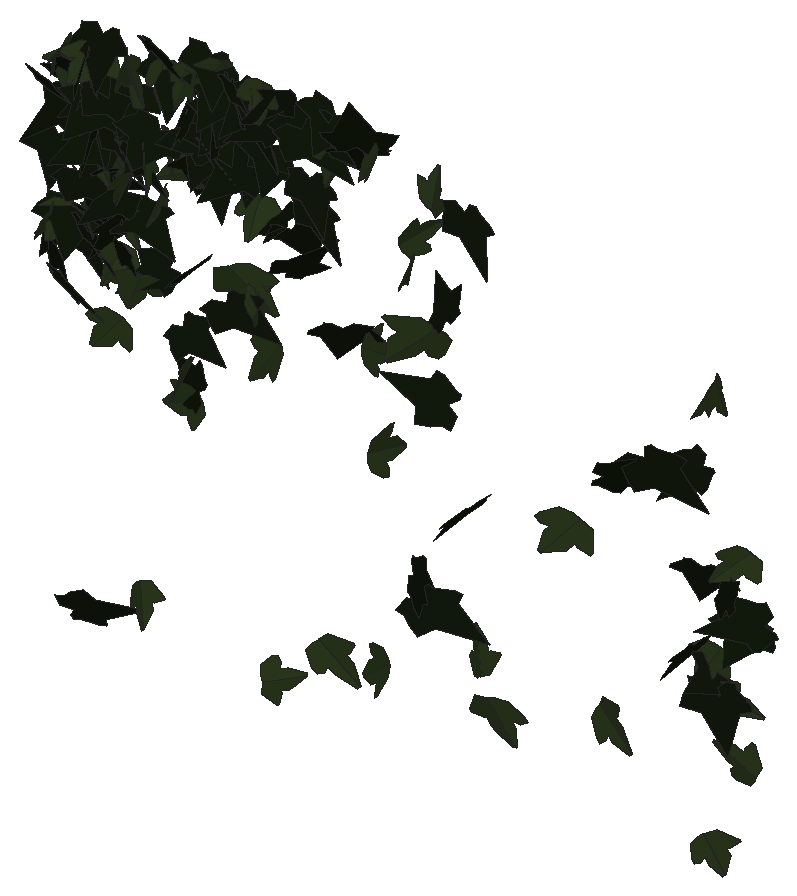
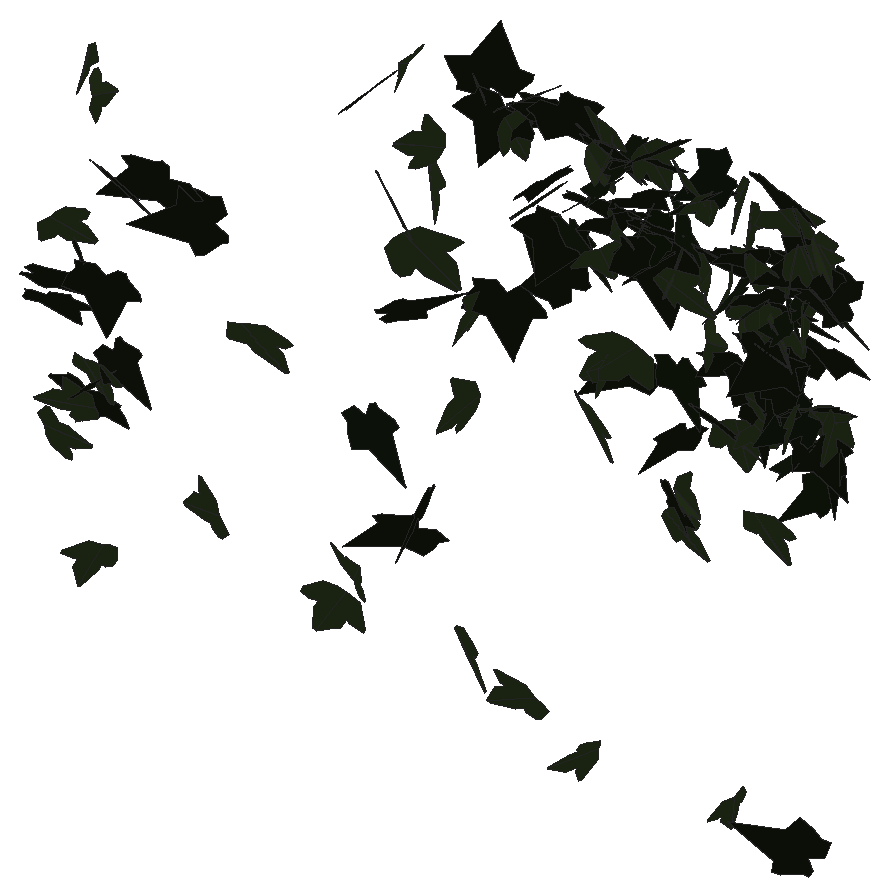
# SketchUp Ruby script. Lengths in inches.
U = 1.inch
M = Sketchup.active_model
def pt(a) = Geom::Point3d.new(a.map { |v| v * U })
def face(e, loops, mat)
  f = e.add_face(loops[0].map { |a| pt(a) })
  loops[1..].each { |l| e.add_face(l.map { |a| pt(a) }).erase! }
  f.material = f.back_material = mat if mat
  f
end
# faces: each face lists its corners as indices into pts; further lists are holes
def faces(e, pts, list, mat = nil) = list.each { |f| face(e, (f[0].is_a?(Array) ? f : [f]).map { |l| l.map { |i| pts[i] } }, mat) }
# xy, xz, yz: faces in a plane at the given z, y or x. An outline is a flat list of corners, or four numbers for a rectangle; further outlines are holes
def ring(l) = l.size == 4 ? [[l[0], l[1]], [l[2], l[1]], [l[2], l[3]], [l[0], l[3]]] : l.each_slice(2).to_a
def flat(e, list, mat, &to3) = list.each { |f| face(e, (f[0].is_a?(Array) ? f : [f]).map { |l| ring(l).map { |u, v| to3.(u, v) } }, mat) }
def xy(e, z, list, mat = nil) = flat(e, list, mat) { |x, y| [x, y, z] }
def xz(e, y, list, mat = nil) = flat(e, list, mat) { |x, z| [x, y, z] }
def yz(e, x, list, mat = nil) = flat(e, list, mat) { |y, z| [x, y, z] }
def lines(e, pts, list) = list.each { |a, b| e.add_line(pt(pts[a]), pt(pts[b])) }
# prism: a flat outline (further loops are holes) pulled along v
def prism(e, loops, v, mat = nil)
  f = face(e, loops, mat); d = Geom::Vector3d.new(v.map { |x| x * U })
  f.pushpull(f.normal.samedirection?(d) ? d.length : -d.length)
end
def box(e, o, s, mat = nil) = prism(e, [[o, [o[0] + s[0], o[1], o[2]], [o[0] + s[0], o[1] + s[1], o[2]], [o[0], o[1] + s[1], o[2]]]], [0, 0, s[2]], mat)
def at(x, y, z, deg = 0) = Geom::Transformation.translation(pt([x, y, z])) * Geom::Transformation.rotation(ORIGIN, Z_AXIS, deg.degrees)
def axes(o, x, y, z) = Geom::Transformation.new([*x, 0, *y, 0, *z, 0, *pt(o).to_a, 1])
def part(name) = M.definitions.add(name)
# library, detail: a bought-in or finely detailed component or shape, given as its bounding box
def library(name, o, s) = part(name).tap { |d| box(d.entities, o, s) }
def detail(e, o, s) = box(e.add_group.entities, o, s)
def put(e, d, t, mat = nil) = e.add_instance(d, t).tap { |i| i.material = mat if mat }
def group(e, t, mat = nil) = e.add_group.tap { |g| g.transformation = t; g.material = mat if mat }.entities
root = M.entities
M.materials.add("1026 AP 7946 SUNNY SIDE UP").color = [254, 231, 186]
M.materials.add("efeu1").color = [18, 25, 13]
M.materials.add("efeu2").color = [43, 57, 29]
c1 = part("ivyleaf_9")
p = [[1.54,2.16,1.25],[1.36,2.04,1.19],[-0.21,0.99,0.68],[-0.71,1.11,0.82],[-0.85,0.86,0.67],[-0.8,0.17,0.21],
  [-0.9,-0.01,0.1],[-0.67,-0.16,-0.02],[-0.08,-0.08,-0.05],[-0.03,-0.6,-0.4],[0.65,-0.88,-0.66],[0.83,-0.6,-0.49],
  [1.29,-0.42,-0.43],[1.8125,-0.07,-0.26],[1.21,0.44,0.15]]
faces(c1.entities,p,[[0,1,2,3,4,5,6,7,8,9,10,11,12,13,14]],"efeu1")
c2 = part("ivyleaf_10")
p = [[0,0.5,-0.03],[-0.0625,2.02,-0.43],[-0.19,2.01,-0.46],[-0.54,1.05,-0.29],[-0.52,0.625,-0.18],[-0.83,0.76,-0.28],
  [-1.16,0.64,-0.33],[-1.15,0.33,-0.24],[-0.77,-0.39,0.02],[-0.3,-0.51,0.16],[0.04,-0.48,0.23],[-0.02,2.01,-0.4375],
  [-0.06,2.01,-0.43],[0.04,-0.49,0.23],[0.67,-0.49,0.14],[1.38,0.36,-0.2],[1.375,0.51,-0.24],[0.81,0.65,-0.19],
  [0.62,0.59,-0.15],[0.6,1.09,-0.28],[0.5,1.23,-0.31]]
faces(c2.entities,p,[[0,1,2,3,4,5,6,7,8,9,10],[11,12,0,13,14,15,16,17,18,19,20]],"efeu2")
put(root,c1,axes([127.99,212.35,274.9],[0.2386,-0.046,-0.27535],[-0.41018,0.05791,-0.16266],[0.11515,0.30161,-0.00889]),"1026 AP 7946 SUNNY SIDE UP")
put(root,c1,axes([127.54,212.61,277.8],[0.30684,-0.18203,0.16089],[0.1912,-0.1,-0.27537],[0.32631,0.22977,0.01006]),"1026 AP 7946 SUNNY SIDE UP")
put(root,c2,axes([127.93,212.35,275.47],[-0.04301,-0.23789,-0.23167],[0.05468,0.22091,-0.2453],[0.51036,-0.04372,0.00676]),"1026 AP 7946 SUNNY SIDE UP")
put(root,c1,axes([128.04,212.64,275.1875],[0.00942,0.23509,-0.17942],[0.0038,-0.17557,-0.24323],[-0.46129,0.00335,-0.00567]),"1026 AP 7946 SUNNY SIDE UP")
put(root,c2,axes([127.98,212.68,278.6],[0.0953,-0.30672,0.00333],[-0.02376,-0.00805,-0.32169],[0.48176,0.06028,-0.01652]),"1026 AP 7946 SUNNY SIDE UP")
put(root,c1,axes([127.89,212.6,276.85],[-0.36333,-0.10161,-0.1693],[0.26317,0.02097,-0.25656],[0.15025,-0.28243,0.03998]),"1026 AP 7946 SUNNY SIDE UP")
put(root,c1,axes([128.22,212.48,277.72],[-0.48161,0.1498,-0.12186],[0.14484,-0.08171,-0.35027],[-0.26381,-0.31833,0.03016]),"1026 AP 7946 SUNNY SIDE UP")
put(root,c2,axes([128.18,212.78,278.42],[-0.26163,-0.24846,0.09229],[-0.01566,-0.10153,-0.30496],[0.41575,-0.16018,0.04659]),"1026 AP 7946 SUNNY SIDE UP")
put(root,c2,axes([128.22,212.47,275.59],[0.38077,0.12339,-0.11725],[-0.14542,-0.07012,-0.27972],[-0.22118,0.25852,-0.01794]),"1026 AP 7946 SUNNY SIDE UP")
put(root,c1,axes([128.08,212.38,274.3],[0.41901,-0.13176,-0.08034],[-0.0798,0.07011,-0.30318],[0.22651,0.26844,0.04181]),"1026 AP 7946 SUNNY SIDE UP")
put(root,c1,axes([127.98,212.57,278.25],[0.44552,0.04071,0.12678],[0.19072,0.0195,-0.29477],[-0.07091,0.3082,0.00374]),"1026 AP 7946 SUNNY SIDE UP")
put(root,c1,axes([128.28,212.52,275.62],[-0.25069,-0.24515,-0.04338],[0.06927,0.01973,-0.29996],[0.38457,-0.16336,0.02575]),"1026 AP 7946 SUNNY SIDE UP")
put(root,c2,axes([128.31,212.62,277.34],[0.11567,-0.29374,0.00492],[0.11757,0.01229,-0.30203],[0.44678,0.07281,0.0782]),"1026 AP 7946 SUNNY SIDE UP")
put(root,c1,axes([128.23,212.84,274.98],[0.17548,-0.27226,0.02357],[0.01504,-0.02248,-0.30326],[0.42956,0.11201,0.00099]),"1026 AP 7946 SUNNY SIDE UP")
put(root,c2,axes([128.53,212.64,278.29],[-0.25269,0.24743,0.11069],[-0.12618,0.07385,-0.30238],[-0.40404,-0.17781,0.02521]),"1026 AP 7946 SUNNY SIDE UP")
put(root,c2,axes([128.51,212.65,275.5625],[-0.16157,0.25366,0.11537],[-0.0912,0.09555,-0.28087],[-0.42542,-0.11683,0.0164]),"1026 AP 7946 SUNNY SIDE UP")
put(root,c1,axes([128.39,212.64,278.77],[-0.21028,0.01901,-0.29032],[0.40213,-0.12447,-0.13435],[-0.18891,-0.28612,0.03716]),"1026 AP 7946 SUNNY SIDE UP")
put(root,c1,axes([128.3125,212.62,275.57],[0.4558,-0.05076,-0.00583],[-0.01034,-0.00643,-0.30311],[0.0796,0.28985,-0.00599]),"1026 AP 7946 SUNNY SIDE UP")
put(root,c1,axes([128.37,212.87,277.28],[0.23794,-0.25749,0.05404],[0.04225,-0.04675,-0.30796],[0.4115,0.15369,0.00037]),"1026 AP 7946 SUNNY SIDE UP")
put(root,c2,axes([128.78,212.49,278.79],[0.40867,0.10648,-0.14054],[-0.18521,-0.07297,-0.289],[-0.20037,0.28461,-0.01951]),"1026 AP 7946 SUNNY SIDE UP")
put(root,c2,axes([128.78,212.74,276.96],[0.2219,-0.26805,-0.04438],[-0.05542,0.02833,-0.31137],[0.4229,0.14436,-0.01751]),"1026 AP 7946 SUNNY SIDE UP")
put(root,c1,axes([128.97,212.5,277.15],[-0.46108,-0.02133,0.05455],[-0.07729,-0.04777,-0.29985],[0.04599,-0.29414,0.04297]),"1026 AP 7946 SUNNY SIDE UP")
put(root,c1,axes([128.83,212.6,277.8125],[-0.33045,-0.19934,0.09583],[-0.05109,-0.10065,-0.29483],[0.34285,-0.20712,0.04843]),"1026 AP 7946 SUNNY SIDE UP")
put(root,c1,axes([128.6875,212.5625,277.375],[-0.22287,0.04578,-0.27231],[0.36202,-0.13325,-0.15159],[-0.21728,-0.26896,0.02675]),"1026 AP 7946 SUNNY SIDE UP")
put(root,c1,axes([128.39,212.52,267.93],[0.15057,-0.04342,0.2928],[0.45115,-0.00847,-0.10088],[0.03453,0.30003,0.04131]),"1026 AP 7946 SUNNY SIDE UP")
put(root,c1,axes([128.55,212.52,275.39],[0.24814,-0.24452,0.05174],[0.01895,-0.05352,-0.29951],[0.3925,0.15717,-0.01825]),"1026 AP 7946 SUNNY SIDE UP")
put(root,c1,axes([128.99,212.54,275.62],[0.16965,-0.14209,0.25963],[-0.22303,0.20943,0.18484],[-0.39776,-0.17804,0.00709]),"1026 AP 7946 SUNNY SIDE UP")
put(root,c1,axes([129.09,212.61,278.11],[-0.47798,0.00001,0.0364],[-0.05531,-0.02867,-0.31195],[0.00519,-0.30468,0.02756]),"1026 AP 7946 SUNNY SIDE UP")
put(root,c1,axes([128.62,212.34,276.51],[-0.02841,-0.10689,-0.29868],[0.17158,0.26886,-0.10777],[0.45362,-0.10839,0.02206]),"1026 AP 7946 SUNNY SIDE UP")
put(root,c2,axes([128.61,212.6,276.89],[0.28998,-0.06078,0.23919],[0.34699,-0.07328,-0.20046],[0.1497,0.28759,0.00133]),"1026 AP 7946 SUNNY SIDE UP")
put(root,c2,axes([129.01,212.75,273.56],[0.41792,-0.07395,-0.12679],[-0.18136,0.04276,-0.28379],[0.13351,0.28958,0.01137]),"1026 AP 7946 SUNNY SIDE UP")
put(root,c1,axes([128.77,212.52,276.375],[0.34241,0.21301,0.15905],[0.17709,0.1039,-0.31319],[-0.37261,0.24513,-0.00269]),"1026 AP 7946 SUNNY SIDE UP")
put(root,c1,axes([128.93,212.51,279.19],[-0.35687,-0.08126,-0.2231],[0.35704,-0.02377,-0.23661],[0.06564,-0.31248,0.07406]),"1026 AP 7946 SUNNY SIDE UP")
put(root,c1,axes([129.01,212.81,277.5],[-0.22148,-0.26899,-0.00087],[0.00897,-0.00376,-0.31275],[0.42286,-0.1408,0.00618]),"1026 AP 7946 SUNNY SIDE UP")
put(root,c2,axes([129.25,212.6,277.1],[-0.46009,-0.05613,0.03196],[-0.03464,-0.0497,-0.3038],[0.09497,-0.29005,0.04406]),"1026 AP 7946 SUNNY SIDE UP")
put(root,c2,axes([129.04,212.83,278.01],[0.44831,-0.06202,0.10589],[0.14973,-0.04594,-0.2999],[0.11573,0.29969,-0.02219]),"1026 AP 7946 SUNNY SIDE UP")
put(root,c1,axes([129.3,212.4375,275.36],[0.27622,-0.02047,-0.2536],[-0.38694,0.01002,-0.1818],[0.03154,0.30216,-0.00937]),"1026 AP 7946 SUNNY SIDE UP")
put(root,c2,axes([129.23,212.625,275.06],[0.1726,0.21273,-0.1807],[-0.12477,-0.1578,-0.24752],[-0.41646,0.13544,-0.00074]),"1026 AP 7946 SUNNY SIDE UP")
put(root,c1,axes([129.03,212.7,277.33],[0.16864,-0.29083,-0.02972],[0.00926,0.03112,-0.31871],[0.4592,0.10618,0.01734]),"1026 AP 7946 SUNNY SIDE UP")
put(root,c1,axes([129.44,212.48,276.35],[-0.46351,0.02819,-0.04096],[0.05495,-0.04903,-0.3018],[-0.05372,-0.2934,0.04472]),"1026 AP 7946 SUNNY SIDE UP")
put(root,c2,axes([129.3,212.625,278.71],[0.10779,-0.26987,-0.16559],[0.05505,0.16854,-0.27781],[0.48959,0.04046,0.06769]),"1026 AP 7946 SUNNY SIDE UP")
put(root,c1,axes([129.28,212.89,278.14],[-0.24342,-0.26367,0.00497],[0.02881,-0.01807,-0.31404],[0.41371,-0.15388,0.02479]),"1026 AP 7946 SUNNY SIDE UP")
put(root,c1,axes([129.47,212.42,275.87],[-0.08769,0.25781,-0.22566],[0.07086,-0.21586,-0.273],[-0.52872,-0.07169,0.00084]),"1026 AP 7946 SUNNY SIDE UP")
put(root,c2,axes([129.13,212.83,275.67],[0.1786,-0.03269,0.2821],[0.37532,-0.13707,-0.11958],[0.21777,0.26305,-0.02527]),"1026 AP 7946 SUNNY SIDE UP")
put(root,c2,axes([129.47,212.52,276.68],[0.02689,-0.30373,0.05021],[0.01116,-0.05014,-0.31366],[0.484,0.01803,0.00444]),"1026 AP 7946 SUNNY SIDE UP")
put(root,c2,axes([129.73,212.48,274.77],[-0.3898,-0.14838,0.07193],[-0.07288,-0.05958,-0.29673],[0.24793,-0.2508,0.02587]),"1026 AP 7946 SUNNY SIDE UP")
put(root,c2,axes([129.58,212.78,268.58],[0.06164,0.29237,-0.07784],[-0.0167,-0.07649,-0.30434],[-0.4752,0.04062,0.0006]),"1026 AP 7946 SUNNY SIDE UP")
put(root,c2,axes([129.73,212.34,278.84],[-0.21135,0.28741,0.08549],[-0.07828,0.0664,-0.32604],[-0.4631,-0.14239,0.0161]),"1026 AP 7946 SUNNY SIDE UP")
put(root,c1,axes([129.61,212.47,277.27],[0.28431,-0.2237,-0.12274],[-0.10458,0.09773,-0.29561],[0.38359,0.19245,0.01038]),"1026 AP 7946 SUNNY SIDE UP")
put(root,c1,axes([129.57,212.59,276.06],[-0.0612,-0.2065,-0.2284],[0.26236,0.17068,-0.19398],[0.39605,-0.14498,0.09321]),"1026 AP 7946 SUNNY SIDE UP")
put(root,c1,axes([130.14,212.74,275.02],[-0.45594,0.07886,-0.00566],[-0.00286,-0.02922,-0.30833],[-0.12432,-0.28855,0.02784]),"1026 AP 7946 SUNNY SIDE UP")
put(root,c2,axes([129.89,212.49,277.24],[-0.06175,0.23853,-0.20952],[0.05414,-0.20182,-0.25021],[-0.49129,-0.05222,-0.00124]),"1026 AP 7946 SUNNY SIDE UP")
put(root,c2,axes([130,212.82,276.35],[-0.08975,0.1631,-0.25348],[-0.06826,-0.25342,-0.16356],[-0.46035,0.00578,0.07367]),"1026 AP 7946 SUNNY SIDE UP")
put(root,c1,axes([130.09,212.55,277.73],[-0.40678,-0.15578,-0.01435],[0.03527,-0.01202,-0.31036],[0.24327,-0.25875,0.021]),"1026 AP 7946 SUNNY SIDE UP")
put(root,c1,axes([129.82,212.6875,279.23],[0.45135,-0.13655,0.00495],[-0.0128,-0.03004,-0.32612],[0.21451,0.28552,-0.02987]),"1026 AP 7946 SUNNY SIDE UP")
put(root,c2,axes([130.04,212.76,278.8],[0.14593,0.28498,-0.06993],[-0.01965,-0.06898,-0.30902],[-0.46082,0.09319,-0.00897]),"1026 AP 7946 SUNNY SIDE UP")
put(root,c2,axes([130.07,212.8,277.52],[-0.21283,0.2009,-0.18028],[0.08526,-0.17268,-0.24685],[-0.41137,-0.13973,0.04211]),"1026 AP 7946 SUNNY SIDE UP")
put(root,c1,axes([130.11,212.91,278.77],[-0.13353,-0.29427,0.02455],[0.00438,-0.02733,-0.31551],[0.46442,-0.08435,0.01004]),"1026 AP 7946 SUNNY SIDE UP")
put(root,c2,axes([130.74,212.85,277.1],[-0.24165,-0.05176,0.2626],[-0.34884,-0.12912,-0.16537],[0.21437,-0.26846,0.02692]),"1026 AP 7946 SUNNY SIDE UP")
put(root,c1,axes([130.61,212.5,277.88],[0.08769,0.08498,0.3436],[0.04648,0.33497,-0.09119],[-0.53847,0.04276,0.04808]),"1026 AP 7946 SUNNY SIDE UP")
put(root,c2,axes([130.59,212.68,278.91],[0.35705,-0.21916,0.01935],[-0.00182,-0.02997,-0.32447],[0.34603,0.22598,-0.02168]),"1026 AP 7946 SUNNY SIDE UP")
put(root,c2,axes([130.9,212.48,272.82],[0.23053,-0.09939,-0.25825],[-0.31554,0.14943,-0.18148],[0.28201,0.24844,0.00806]),"1026 AP 7946 SUNNY SIDE UP")
put(root,c2,axes([130.68,212.61,273.39],[0.16454,-0.23069,0.18315],[0.08703,-0.17113,-0.2614],[0.4509,0.11721,-0.01639]),"1026 AP 7946 SUNNY SIDE UP")
put(root,c1,axes([131.04,212.45,273.11],[-0.24552,0.11226,-0.24567],[-0.38367,0.0451,0.18623],[0.1591,0.28199,0.06997]),"1026 AP 7946 SUNNY SIDE UP")
put(root,c2,axes([130.72,212.86,277.03],[-0.14901,0.24243,0.15972],[0.10611,-0.13846,0.26711],[0.43866,0.11584,-0.01036]),"1026 AP 7946 SUNNY SIDE UP")
put(root,c1,axes([131.1,212.71,277.84],[-0.40482,0.08649,0.13841],[-0.2316,-0.03197,-0.27073],[-0.09573,-0.28841,0.06966]),"1026 AP 7946 SUNNY SIDE UP")
put(root,c1,axes([130.91,212.42,275.41],[-0.08129,0.29429,-0.03334],[0.01593,-0.03277,-0.30798],[-0.46555,-0.05251,-0.00472]),"1026 AP 7946 SUNNY SIDE UP")
put(root,c1,axes([131.0625,212.7,277.45],[0.2267,0.29437,-0.16466],[-0.09493,-0.15017,-0.33837],[-0.51935,0.15594,-0.01002]),"1026 AP 7946 SUNNY SIDE UP")
put(root,c1,axes([130.85,212.35,274.29],[0.10184,-0.16027,-0.25801],[-0.08016,0.2456,-0.17469],[0.45939,0.07838,0.02671]),"1026 AP 7946 SUNNY SIDE UP")
put(root,c2,axes([131.11,212.85,279.2],[-0.16476,-0.26485,0.11791],[-0.01694,-0.11967,-0.29233],[0.4543,-0.10051,0.03186]),"1026 AP 7946 SUNNY SIDE UP")
put(root,c1,axes([130.97,212.91,279.32],[-0.0851,-0.30283,0.03364],[0.0093,-0.03595,-0.31688],[0.47913,-0.05309,0.01212]),"1026 AP 7946 SUNNY SIDE UP")
put(root,c1,axes([131.13,212.6875,277.84],[-0.40091,-0.12565,-0.10832],[0.18875,-0.01276,-0.28618],[0.17428,-0.27523,0.06077]),"1026 AP 7946 SUNNY SIDE UP")
put(root,c1,axes([131.12,212.8125,277.25],[-0.01663,-0.30447,0.02122],[-0.00646,-0.0222,-0.31396],[0.47999,-0.01085,-0.00349]),"1026 AP 7946 SUNNY SIDE UP")
put(root,c1,axes([131.04,212.62,277.71],[0.38641,-0.19039,0.0366],[0.0205,-0.04274,-0.31942],[0.30417,0.24475,-0.02496]),"1026 AP 7946 SUNNY SIDE UP")
put(root,c1,axes([131.38,212.83,278.93],[-0.37233,-0.19213,0.00309],[0.02224,-0.0239,-0.313],[0.30136,-0.23561,0.02692]),"1026 AP 7946 SUNNY SIDE UP")
put(root,c1,axes([131.39,212.89,278.375],[-0.28893,-0.23198,0.07906],[-0.05144,-0.07346,-0.30465],[0.38141,-0.18564,0.01881]),"1026 AP 7946 SUNNY SIDE UP")
put(root,c1,axes([131.18,212.88,278.03],[0.13832,-0.11525,-0.27788],[0.31252,-0.18277,0.14651],[-0.33793,-0.2162,0.02175]),"1026 AP 7946 SUNNY SIDE UP")
put(root,c1,axes([131.51,212.82,278.98],[0.25183,-0.26002,0.02195],[0.0234,-0.01759,-0.31469],[0.40975,0.16081,0.00448]),"1026 AP 7946 SUNNY SIDE UP")
put(root,c1,axes([132.01,212.5,277.74],[-0.49214,-0.02006,-0.02789],[0.045,-0.0268,-0.32192],[0.02769,-0.313,0.0275]),"1026 AP 7946 SUNNY SIDE UP")
put(root,c2,axes([131.74,212.66,275.49],[-0.46413,-0.05384,-0.21885],[0.33845,-0.007,-0.30676],[0.06224,-0.36342,0.03616]),"1026 AP 7946 SUNNY SIDE UP")
put(root,c1,axes([132.08,212.78,278.97],[-0.47182,-0.02701,-0.06739],[0.10729,-0.03724,-0.30753],[0.0287,-0.30481,0.04172]),"1026 AP 7946 SUNNY SIDE UP")
put(root,c2,axes([131.72,212.82,277.6875],[0.3008,-0.08753,0.23033],[0.29151,-0.12879,-0.21564],[0.24105,0.26499,-0.02664]),"1026 AP 7946 SUNNY SIDE UP")
put(root,c1,axes([131.93,212.84,277.8],[-0.18788,-0.28286,-0.00493],[0.01204,0.00022,-0.31625],[0.44464,-0.11953,0.00648]),"1026 AP 7946 SUNNY SIDE UP")
put(root,c2,axes([131.93,212.8,278.98],[-0.0872,0.23128,-0.19637],[0.05168,-0.18933,-0.24593],[-0.46974,-0.06376,0.00939]),"1026 AP 7946 SUNNY SIDE UP")
put(root,c1,axes([131.81,212.32,275.1],[-0.00596,-0.10008,-0.29943],[0.11996,0.28069,-0.09915],[0.46737,-0.07332,0.02163]),"1026 AP 7946 SUNNY SIDE UP")
put(root,c1,axes([131.86,212.87,278.46],[0.18004,-0.27999,0.0594],[0.02411,-0.05772,-0.31187],[0.44936,0.11528,-0.00707]),"1026 AP 7946 SUNNY SIDE UP")
put(root,c2,axes([132.15,212.87,278.8],[0.04648,-0.28859,0.10377],[-0.0034,-0.10304,-0.29921],[0.48147,0.02713,-0.01213]),"1026 AP 7946 SUNNY SIDE UP")
put(root,c2,axes([132.19,212.53,275.02],[0.0439,0.10049,-0.30666],[0.0501,0.29697,0.10789],[0.49232,-0.03918,0.01637]),"1026 AP 7946 SUNNY SIDE UP")
put(root,c1,axes([132.22,212.86,278.03],[-0.40748,-0.15099,-0.06976],[0.14153,-0.02485,-0.30174],[0.21769,-0.26647,0.0656]),"1026 AP 7946 SUNNY SIDE UP")
put(root,c2,axes([132.21,212.625,277.03],[0.24233,0.23783,-0.12051],[-0.08248,-0.10686,-0.29227],[-0.40947,0.16228,-0.01244]),"1026 AP 7946 SUNNY SIDE UP")
put(root,c2,axes([132.22,212.63,279.23],[0.42788,-0.12238,0.077],[0.09836,-0.04462,-0.30727],[0.20353,0.27883,-0.01338]),"1026 AP 7946 SUNNY SIDE UP")
put(root,c2,axes([132.4375,212.69,274.27],[0.37718,-0.27248,-0.08313],[-0.11473,0.04091,-0.3727],[0.43115,0.24926,-0.02645]),"1026 AP 7946 SUNNY SIDE UP")
put(root,c1,axes([132.6875,212.45,278.89],[-0.42814,0.14758,-0.00802],[-0.00662,-0.02581,-0.3182],[-0.23235,-0.2712,0.02384]),"1026 AP 7946 SUNNY SIDE UP")
put(root,c1,axes([132.36,212.79,277.98],[-0.10995,-0.26936,0.13799],[-0.00382,-0.13857,-0.28592],[0.47408,-0.06359,0.0297]),"1026 AP 7946 SUNNY SIDE UP")
put(root,c1,axes([132.97,212.4,277.07],[-0.23451,0.26882,0.01624],[-0.03593,0.00358,-0.31612],[-0.42175,-0.14977,0.0179]),"1026 AP 7946 SUNNY SIDE UP")
put(root,c1,axes([133,212.61,279.24],[0.04097,0.08317,-0.30941],[-0.26756,-0.24926,-0.08764],[-0.4114,0.1704,0.02619]),"1026 AP 7946 SUNNY SIDE UP")
put(root,c2,axes([132.65,212.37,268.13],[0.08025,-0.06743,-0.31215],[0.24775,0.26978,-0.03297],[0.41986,-0.1463,0.07912]),"1026 AP 7946 SUNNY SIDE UP")
put(root,c1,axes([133.15,212.375,276.97],[0.37703,0.18975,-0.04615],[-0.02924,-0.05013,-0.31403],[-0.30556,0.23893,-0.02689]),"1026 AP 7946 SUNNY SIDE UP")
put(root,c1,axes([133,212.45,276.11],[0.3312,0.23716,0.03298],[-0.05768,-0.00834,0.32595],[0.37156,-0.21269,0.0212]),"1026 AP 7946 SUNNY SIDE UP")
put(root,c1,axes([133.32,212.62,277.875],[0.0185,-0.30912,-0.03279],[-0.01298,0.02977,-0.31843],[0.48819,0.0125,-0.00722]),"1026 AP 7946 SUNNY SIDE UP")
put(root,c1,axes([133.15,212.47,279.0625],[0.06575,-0.15404,-0.27872],[0.32008,0.2191,-0.09513],[0.36882,-0.16269,0.13225]),"1026 AP 7946 SUNNY SIDE UP")
put(root,c1,axes([133.43,212.54,277.49],[0.13045,-0.30943,-0.03813],[0.01305,0.03867,-0.32929],[0.48953,0.08143,0.01894]),"1026 AP 7946 SUNNY SIDE UP")
put(root,c1,axes([133.37,212.41,278.9375],[-0.00495,-0.20042,-0.24959],[0.24591,0.20801,-0.17899],[0.42733,-0.12202,0.10011]),"1026 AP 7946 SUNNY SIDE UP")
put(root,c1,axes([133.68,212.8,279.1875],[-0.20367,-0.24956,0.14229],[-0.00859,-0.151,-0.28432],[0.4495,-0.11596,0.05904]),"1026 AP 7946 SUNNY SIDE UP")
put(root,c2,axes([133.9,212.69,278.62],[-0.07107,-0.27731,0.14063],[0.05059,-0.14299,-0.28583],[0.48448,-0.02575,0.05048]),"1026 AP 7946 SUNNY SIDE UP")
put(root,c2,axes([133.6,212.6875,268.91],[0.28581,0.06099,0.26352],[0.40563,0.01684,-0.19314],[-0.0775,0.31307,-0.03905]),"1026 AP 7946 SUNNY SIDE UP")
put(root,c1,axes([134.14,212.58,278.79],[0.2912,0.25346,-0.00007],[0.01687,-0.0097,-0.32311],[-0.3982,0.18495,-0.01373]),"1026 AP 7946 SUNNY SIDE UP")
put(root,c1,axes([134.25,212.35,275.46],[0.23761,0.24629,-0.1335],[-0.10655,-0.1121,-0.29833],[-0.42549,0.16561,0.00015]),"1026 AP 7946 SUNNY SIDE UP")
put(root,c1,axes([134.48,212.43,279.06],[0.39385,0.08383,0.202],[-0.31761,-0.00147,0.2671],[0.10536,-0.3178,0.05006]),"1026 AP 7946 SUNNY SIDE UP")
put(root,c2,axes([134.7,212.5,275.16],[-0.0709,0.16965,0.2952],[-0.11641,0.27583,-0.17922],[-0.50918,-0.08668,-0.00014]),"1026 AP 7946 SUNNY SIDE UP")
put(root,c2,axes([134.8,212.42,278.99],[0.23509,-0.28435,-0.07534],[-0.05633,0.06196,-0.33058],[0.45758,0.15372,-0.00199]),"1026 AP 7946 SUNNY SIDE UP")
put(root,c2,axes([135.07,212.37,269.24],[0.20891,-0.23676,-0.2348],[-0.212,0.18334,-0.27775],[0.46965,0.18807,-0.02093]),"1026 AP 7946 SUNNY SIDE UP")
put(root,c2,axes([135.01,212.33,273.35],[0.01544,0.07379,0.38232],[-0.12677,0.36269,-0.07006],[-0.58064,-0.07722,0.02546]),"1026 AP 7946 SUNNY SIDE UP")
put(root,c2,axes([135.5625,212.5,277.15],[0.12208,-0.29535,-0.15167],[-0.01913,0.14686,-0.31284],[0.51738,0.07512,0.02422]),"1026 AP 7946 SUNNY SIDE UP")
put(root,c2,axes([135.86,212.57,275.84],[-0.36516,-0.1763,0.25734],[-0.2571,-0.19491,-0.29827],[0.40775,-0.28078,0.04239]),"1026 AP 7946 SUNNY SIDE UP")
put(root,c2,axes([135.61,212.46,277.59],[0.01025,-0.12684,0.31021],[0.00872,0.3019,0.13234],[-0.51474,0.00259,0.00842]),"1026 AP 7946 SUNNY SIDE UP")
put(root,c1,axes([135.9,212.23,271.33],[0.21786,-0.1184,-0.31716],[-0.33606,0.22117,-0.18583],[0.39376,0.25426,0.01688]),"1026 AP 7946 SUNNY SIDE UP")
put(root,c1,axes([136.22,212.63,274.6],[-0.19165,-0.27724,-0.12247],[-0.07529,-0.10709,0.31136],[-0.46732,0.13095,0.00006]),"1026 AP 7946 SUNNY SIDE UP")
put(root,c1,axes([136.35,212.47,276.37],[0.00727,0.12632,0.32682],[-0.08811,0.31252,-0.12582],[-0.52857,-0.05036,0.02547]),"1026 AP 7946 SUNNY SIDE UP")
put(root,c2,axes([136.24,212.22,278.69],[0.0755,0.16571,-0.27886],[-0.01681,0.27539,0.17274],[0.50003,-0.01576,0.04791]),"1026 AP 7946 SUNNY SIDE UP")
put(root,c1,axes([136.02,212.35,270.82],[0.08294,-0.12494,-0.30697],[0.19377,0.28616,-0.09971],[0.46854,-0.09623,0.09557]),"1026 AP 7946 SUNNY SIDE UP")
put(root,c1,axes([136.64,212.71,272.66],[-0.15862,0.30015,-0.13094],[0.05041,-0.12506,-0.32681],[-0.5111,-0.10549,0.0084]),"1026 AP 7946 SUNNY SIDE UP")
put(root,c1,axes([136.59,212.71,278.33],[0.09904,-0.34593,-0.01629],[-0.01498,0.01233,-0.36208],[0.54416,0.0633,-0.007]),"1026 AP 7946 SUNNY SIDE UP")
put(root,c2,axes([136.98,212.66,269.79],[0.35942,-0.11724,0.21313],[-0.26276,0.12626,0.2638],[-0.2673,-0.28176,0.02727]),"1026 AP 7946 SUNNY SIDE UP")
put(root,c2,axes([137.37,212.51,269.2],[-0.48565,0.03436,-0.11359],[0.16426,-0.05242,-0.31802],[-0.07812,-0.3238,0.03746]),"1026 AP 7946 SUNNY SIDE UP")
put(root,c2,axes([138.98,212.5625,273.25],[0.47999,-0.03236,-0.14333],[-0.22232,-0.02488,-0.31419],[0.0299,0.33447,-0.03525]),"1026 AP 7946 SUNNY SIDE UP")
put(root,c2,axes([139.72,212.53,269.86],[0.19013,-0.03906,0.33711],[0.48511,-0.10981,-0.1315],[0.18318,0.33134,-0.00166]),"1026 AP 7946 SUNNY SIDE UP")
put(root,c1,axes([139.98,212.3,274.66],[0.30243,0.08071,0.27233],[0.38257,0.10219,-0.21428],[-0.20476,0.31014,0.00187]),"1026 AP 7946 SUNNY SIDE UP")
put(root,c1,axes([140.75,212.4,275.19],[-0.03144,-0.07043,-0.34739],[0.37346,0.24129,-0.06509],[0.39149,-0.23583,0.0342]),"1026 AP 7946 SUNNY SIDE UP")
put(root,c1,axes([141.58,212.8,275.18],[-0.45024,0.07165,-0.06623],[0.08683,-0.04454,-0.30285],[-0.1245,-0.29016,0.02829]),"1026 AP 7946 SUNNY SIDE UP")
put(root,c1,axes([141.6875,212.46,271.9],[-0.14493,0.23589,-0.16284],[0.07571,-0.15222,-0.26163],[-0.44121,-0.10361,0.00859]),"1026 AP 7946 SUNNY SIDE UP")
put(root,c1,axes([141.6875,212.71,273.3],[0.32257,0.13625,-0.16468],[-0.18483,-0.11199,-0.25319],[-0.27481,0.23525,-0.02301]),"1026 AP 7946 SUNNY SIDE UP")
put(root,c2,axes([141.68,212.96,276.58],[-0.08058,0.1093,-0.28877],[-0.08204,-0.28388,-0.10564],[-0.46684,0.03102,0.06841]),"1026 AP 7946 SUNNY SIDE UP")
put(root,c2,axes([141.91,212.75,271.71],[0.4192,-0.10416,-0.05792],[-0.09307,0.001,-0.29412],[0.16067,0.27234,-0.01924]),"1026 AP 7946 SUNNY SIDE UP")
put(root,c1,axes([142.01,212.81,271.31],[-0.20046,-0.14,0.21591],[-0.13039,-0.1994,-0.18964],[0.37534,-0.14404,0.04943]),"1026 AP 7946 SUNNY SIDE UP")
put(root,c2,axes([142.08,212.6,276.95],[0.10403,-0.27032,-0.09252],[0.12384,0.10451,-0.26826],[0.42965,0.03533,0.09973]),"1026 AP 7946 SUNNY SIDE UP")
put(root,c2,axes([142.1,212.37,268.3],[0.21681,0.24631,0.11426],[0.03397,0.11251,-0.28807],[-0.4225,0.13545,0.03547]),"1026 AP 7946 SUNNY SIDE UP")
put(root,c1,axes([142.12,212.58,271.14],[-0.33548,-0.11567,-0.25584],[0.37352,0.07703,-0.2474],[0.2127,-0.3177,0.03094]),"1026 AP 7946 SUNNY SIDE UP")
put(root,c2,axes([142.1,212.71,270.98],[0.08832,0.0394,0.28444],[0.40605,0.09843,-0.06807],[-0.16472,0.26377,-0.01529]),"1026 AP 7946 SUNNY SIDE UP")
put(root,c1,axes([142.63,212.17,273.14],[0.08714,-0.00034,0.33376],[-0.02497,0.32829,0.00507],[-0.50882,-0.01617,0.05691]),"1026 AP 7946 SUNNY SIDE UP")
put(root,c2,axes([142.68,212.58,273.89],[0.23862,0.13817,-0.21922],[-0.25793,-0.13693,-0.21213],[-0.30571,0.22338,0.00786]),"1026 AP 7946 SUNNY SIDE UP")
put(root,c2,axes([143.01,212.32,270.05],[0.1477,0.01764,0.30749],[-0.46699,0.04078,0.09407],[-0.053,-0.31014,0.02801]),"1026 AP 7946 SUNNY SIDE UP")
put(root,c1,axes([142.79,212.68,272.59],[-0.39512,-0.13969,-0.03709],[0.06766,-0.00523,-0.29506],[0.21618,-0.25368,0.02457]),"1026 AP 7946 SUNNY SIDE UP")
put(root,c1,axes([143.12,212.52,272.78],[-0.40709,-0.00427,0.15436],[-0.23313,-0.03705,-0.26518],[0.03495,-0.29684,0.02911]),"1026 AP 7946 SUNNY SIDE UP")
